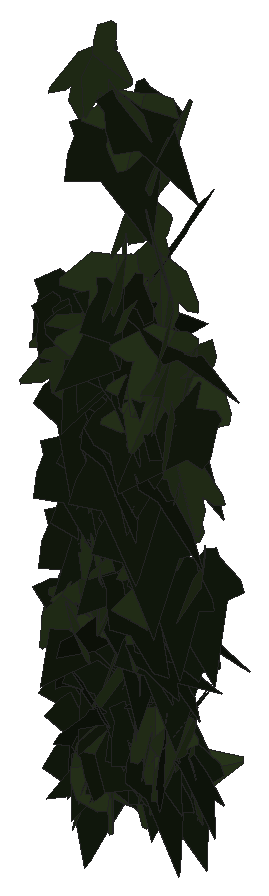
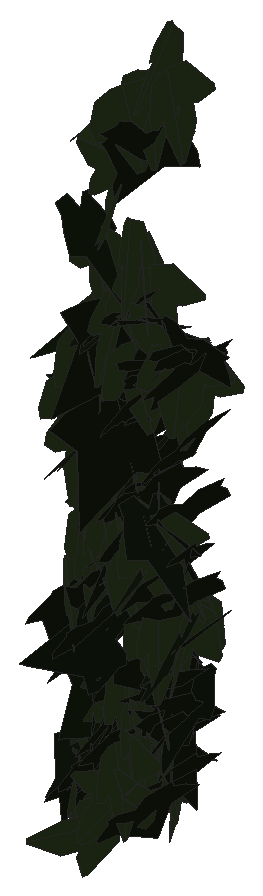
# SketchUp Ruby script. Lengths in inches.
U = 1.inch
M = Sketchup.active_model
def pt(a) = Geom::Point3d.new(a.map { |v| v * U })
def face(e, loops, mat)
  f = e.add_face(loops[0].map { |a| pt(a) })
  loops[1..].each { |l| e.add_face(l.map { |a| pt(a) }).erase! }
  f.material = f.back_material = mat if mat
  f
end
# faces: each face lists its corners as indices into pts; further lists are holes
def faces(e, pts, list, mat = nil) = list.each { |f| face(e, (f[0].is_a?(Array) ? f : [f]).map { |l| l.map { |i| pts[i] } }, mat) }
# xy, xz, yz: faces in a plane at the given z, y or x. An outline is a flat list of corners, or four numbers for a rectangle; further outlines are holes
def ring(l) = l.size == 4 ? [[l[0], l[1]], [l[2], l[1]], [l[2], l[3]], [l[0], l[3]]] : l.each_slice(2).to_a
def flat(e, list, mat, &to3) = list.each { |f| face(e, (f[0].is_a?(Array) ? f : [f]).map { |l| ring(l).map { |u, v| to3.(u, v) } }, mat) }
def xy(e, z, list, mat = nil) = flat(e, list, mat) { |x, y| [x, y, z] }
def xz(e, y, list, mat = nil) = flat(e, list, mat) { |x, z| [x, y, z] }
def yz(e, x, list, mat = nil) = flat(e, list, mat) { |y, z| [x, y, z] }
def lines(e, pts, list) = list.each { |a, b| e.add_line(pt(pts[a]), pt(pts[b])) }
# prism: a flat outline (further loops are holes) pulled along v
def prism(e, loops, v, mat = nil)
  f = face(e, loops, mat); d = Geom::Vector3d.new(v.map { |x| x * U })
  f.pushpull(f.normal.samedirection?(d) ? d.length : -d.length)
end
def box(e, o, s, mat = nil) = prism(e, [[o, [o[0] + s[0], o[1], o[2]], [o[0] + s[0], o[1] + s[1], o[2]], [o[0], o[1] + s[1], o[2]]]], [0, 0, s[2]], mat)
def at(x, y, z, deg = 0) = Geom::Transformation.translation(pt([x, y, z])) * Geom::Transformation.rotation(ORIGIN, Z_AXIS, deg.degrees)
def axes(o, x, y, z) = Geom::Transformation.new([*x, 0, *y, 0, *z, 0, *pt(o).to_a, 1])
def part(name) = M.definitions.add(name)
# library, detail: a bought-in or finely detailed component or shape, given as its bounding box
def library(name, o, s) = part(name).tap { |d| box(d.entities, o, s) }
def detail(e, o, s) = box(e.add_group.entities, o, s)
def put(e, d, t, mat = nil) = e.add_instance(d, t).tap { |i| i.material = mat if mat }
def group(e, t, mat = nil) = e.add_group.tap { |g| g.transformation = t; g.material = mat if mat }.entities
root = M.entities
M.materials.add("efeu1").color = [18, 25, 13]
M.materials.add("efeu2").color = [43, 57, 29]
c1 = part("ivyleaf_9")
p = [[1.54,2.16,1.25],[1.36,2.04,1.19],[-0.21,0.99,0.68],[-0.71,1.11,0.82],[-0.85,0.86,0.67],[-0.8,0.17,0.21],
  [-0.9,-0.01,0.1],[-0.67,-0.16,-0.02],[-0.08,-0.08,-0.05],[-0.03,-0.6,-0.4],[0.65,-0.88,-0.66],[0.83,-0.6,-0.49],
  [1.29,-0.42,-0.43],[1.8125,-0.07,-0.26],[1.21,0.44,0.15]]
faces(c1.entities,p,[[0,1,2,3,4,5,6,7,8,9,10,11,12,13,14]],"efeu1")
c2 = part("ivyleaf_10")
p = [[0,0.5,-0.03],[-0.0625,2.02,-0.43],[-0.19,2.01,-0.46],[-0.54,1.05,-0.29],[-0.52,0.625,-0.18],[-0.83,0.76,-0.28],
  [-1.16,0.64,-0.33],[-1.15,0.33,-0.24],[-0.77,-0.39,0.02],[-0.3,-0.51,0.16],[0.04,-0.48,0.23],[-0.02,2.01,-0.4375],
  [-0.06,2.01,-0.43],[0.04,-0.49,0.23],[0.67,-0.49,0.14],[1.38,0.36,-0.2],[1.375,0.51,-0.24],[0.81,0.65,-0.19],
  [0.62,0.59,-0.15],[0.6,1.09,-0.28],[0.5,1.23,-0.31]]
faces(c2.entities,p,[[0,1,2,3,4,5,6,7,8,9,10],[11,12,0,13,14,15,16,17,18,19,20]],"efeu2")
put(root,c1,axes([23.24,224.17,226.21],[0.01852,-0.47839,-0.14422],[0.05699,0.1454,-0.47499],[0.4964,0.00116,0.05991]))
put(root,c1,axes([23.24,223.85,229.43],[0.14146,-0.43172,-0.20881],[-0.01146,0.2146,-0.45146],[0.47943,0.13252,0.05082]))
put(root,c2,axes([23.55,224.25,227],[-0.25393,-0.41914,0.09918],[-0.03559,-0.09433,-0.48973],[0.42925,-0.25578,0.01808]))
put(root,c2,axes([23.51,223.72,229.37],[-0.33051,-0.37137,-0.05331],[0.03036,0.04434,-0.4971],[0.37395,-0.33184,-0.00676]))
put(root,c1,axes([23.65,224.1875,227.26],[-0.22817,0.42863,-0.11921],[0.05776,-0.1043,-0.48558],[-0.44114,-0.23536,-0.00191]))
put(root,c2,axes([23.59,223.46,225.42],[-0.24049,0.29469,0.32453],[-0.19564,0.2591,-0.38025],[-0.39229,-0.30987,-0.00932]))
put(root,c2,axes([23.53,223.45,229.08],[-0.24872,-0.425,-0.08671],[0.0322,0.08159,-0.49225],[0.43255,-0.25044,-0.01322]))
put(root,c1,axes([23.4,224.75,223.26],[-0.10413,-0.48705,0.04399],[0.00115,-0.04522,-0.49795],[0.48903,-0.1036,0.01054]))
put(root,c2,axes([23.5625,224.08,225.625],[-0.01759,-0.48134,-0.13418],[0.0025,0.13418,-0.48165],[0.49968,-0.01761,-0.00231]))
put(root,c1,axes([23.26,224.1875,225.36],[0.28805,-0.40263,0.07012],[0.04317,-0.05533,-0.49505],[0.4064,0.29125,0.00288]))
put(root,c1,axes([23.37,223.88,227.35],[0.02844,-0.48257,-0.12776],[0.02053,0.12899,-0.48264],[0.49877,0.0222,0.02715]))
put(root,c1,axes([23.49,223.9,225.15],[-0.17656,-0.37444,0.28039],[-0.00324,-0.29872,-0.40095],[0.46778,-0.1434,0.10306]))
put(root,c1,axes([23.4,224.26,226.5],[-0.00186,-0.49802,0.04444],[0.00764,-0.04446,-0.49796],[0.49994,-0.00118,0.00777]))
put(root,c1,axes([23.54,223.38,224.59],[0.4182,-0.00765,-0.27395],[-0.2734,0.02299,-0.418],[0.01899,0.49941,0.01504]))
put(root,c1,axes([23.43,223.9,228.16],[-0.03232,-0.47664,0.14756],[0.01853,-0.14891,-0.47695],[0.49861,-0.02537,0.02729]))
put(root,c1,axes([23.34,223.83,229.78],[-0.18094,-0.25094,-0.3928],[0.35625,0.19726,-0.29013],[0.30057,-0.38486,0.10741]))
put(root,c2,axes([23.53,223.67,225.57],[-0.40171,-0.20217,-0.21854],[0.19322,0.10218,-0.44969],[0.22649,-0.44574,-0.00397]))
put(root,c2,axes([23.55,223.41,225.58],[-0.15429,-0.34275,-0.32972],[0.16956,0.28421,-0.3748],[0.44435,-0.22747,0.02853]))
put(root,c2,axes([23.7,223.66,233.27],[-0.02801,-0.49921,-0.00258],[0.00132,0.00251,-0.49999],[0.49921,-0.02802,0.00118]))
put(root,c2,axes([24.01,223.32,226.09],[-0.16196,0.09948,0.46246],[-0.45935,0.0837,-0.17887],[-0.113,-0.4828,0.06428]))
put(root,c2,axes([23.74,224.69,223.8],[-0.02515,-0.49692,-0.04936],[0.00039,0.04941,-0.49755],[0.49937,-0.02507,-0.0021]))
put(root,c2,axes([23.74,223.79,229.19],[-0.08688,-0.38848,0.30254],[0.04447,-0.31215,-0.38805],[0.49038,-0.04052,0.08879]))
put(root,c1,axes([23.71,223.98,229.24],[-0.24102,-0.43189,0.07332],[-0.01861,-0.07352,-0.49421],[0.43768,-0.24096,0.01937]))
put(root,c2,axes([23.84,223.82,225.56],[-0.26227,-0.37632,0.199],[-0.04535,-0.20771,-0.45255],[0.42327,-0.25543,0.07481]))
put(root,c1,axes([23.7,224.02,224.25],[-0.25181,-0.42707,-0.06482],[0.02996,0.05758,-0.49577],[0.43093,-0.25356,-0.00341]))
put(root,c1,axes([23.77,224.01,229.38],[-0.32089,-0.38306,0.01712],[0.01537,-0.03516,-0.49853],[0.38314,-0.31942,0.03434]))
put(root,c2,axes([23.73,223.85,227.43],[0.22699,-0.4381,-0.0809],[0.05522,0.11776,-0.48279],[0.44207,0.21024,0.10184]))
put(root,c2,axes([23.83,223.42,223.23],[0.15185,-0.37063,-0.29928],[-0.05859,0.2972,-0.39779],[0.47277,0.15588,0.04683]))
put(root,c1,axes([23.93,223.95,226.85],[-0.48859,-0.08267,-0.06669],[0.06554,0.01243,-0.49553],[0.08358,-0.49296,-0.00131]))
put(root,c2,axes([23.8,223.96,224.73],[0.28446,-0.41105,-0.01112],[-0.00679,0.00882,-0.49988],[0.41114,0.28454,-0.00057]))
put(root,c2,axes([23.81,223.8125,223.18],[0.13341,0.08655,0.47404],[-0.11472,0.48343,-0.05597],[-0.46802,-0.09383,0.14885]))
put(root,c1,axes([23.69,223.88,223.18],[-0.07894,-0.48965,0.06333],[0.00504,-0.06493,-0.49574],[0.4937,-0.07763,0.01519]))
put(root,c1,axes([23.66,223.34,224.78],[0.1659,0.17976,0.43607],[0.29169,0.32417,-0.24461],[-0.37067,0.33556,0.00269]))
put(root,c1,axes([23.8,224.16,224.56],[-0.20673,-0.44107,0.11276],[-0.01634,-0.11657,-0.48595],[0.45497,-0.20461,0.03378]))
put(root,c2,axes([23.89,224.18,224.16],[0.07753,-0.484,-0.09867],[0.00047,0.09995,-0.48991],[0.49395,0.07587,0.01595]))
put(root,c1,axes([23.59,224.3125,226.57],[0.23022,-0.43888,0.06621],[0.03144,-0.05827,-0.4956],[0.44273,0.23235,0.00077]))
put(root,c1,axes([23.83,223.92,223.83],[-0.21512,-0.44706,0.06212],[-0.01064,-0.06377,-0.4958],[0.45123,-0.21464,0.01792]))
put(root,c1,axes([23.79,224.1,227.53],[-0.11794,-0.48584,0.00688],[0.00196,-0.00755,-0.49994],[0.48589,-0.1179,0.00369]))
put(root,c2,axes([23.98,224.15,226.4],[-0.0767,-0.44083,0.22313],[-0.02489,-0.22206,-0.44729],[0.49346,-0.07972,0.01212]))
put(root,c2,axes([23.66,224.66,223.37],[0.29172,0.26364,0.30886],[0.22413,0.21259,-0.39316],[-0.33863,0.36783,0.00585]))
put(root,c2,axes([23.97,224.28,224.71],[-0.01009,-0.4981,-0.04237],[0.01138,0.04214,-0.49809],[0.49977,-0.01102,0.01049]))
put(root,c2,axes([24.01,223.98,229.31],[-0.25807,-0.41989,0.08422],[-0.01257,-0.09086,-0.49152],[0.42807,-0.25581,0.03634]))
put(root,c1,axes([24.08,223.54,224.01],[-0.00017,0.39321,-0.30885],[-0.0053,-0.30883,-0.39319],[-0.49997,0.00314,0.00428]))
put(root,c2,axes([23.91,224.13,227.72],[0.27907,-0.41271,0.04229],[0.04637,-0.01962,-0.49746],[0.41227,0.28158,0.02732]))
put(root,c2,axes([23.71,223.86,223.27],[0.30792,-0.18995,0.34511],[0.31552,-0.14336,-0.36041],[0.23587,0.43974,0.03158]))
put(root,c2,axes([24.02,223.74,230.31],[-0.36858,-0.33496,0.04412],[0.03383,-0.10156,-0.48841],[0.33616,-0.35705,0.09754]))
put(root,c2,axes([24.03,224.08,231.12],[0.0932,-0.41518,-0.26257],[-0.02221,0.26342,-0.4244],[0.49073,0.09077,0.03066]))
put(root,c2,axes([23.99,223.2,223.45],[-0.0343,0.1325,0.4809],[-0.07733,0.4748,-0.13633],[-0.49279,-0.08373,-0.01208]))
put(root,c2,axes([24.01,223.9,224.48],[0.12746,-0.47403,0.09514],[0.02879,-0.09078,-0.49085],[0.48262,0.1306,0.00416]))
put(root,c1,axes([23.84,224.36,224.06],[0.07537,-0.44893,-0.20683],[-0.00564,0.20843,-0.45445],[0.49426,0.07083,0.02636]))
put(root,c1,axes([23.86,223.6,223.64],[0.2934,-0.3144,-0.25509],[-0.12723,0.22747,-0.42669],[0.38436,0.31529,0.05348]))
put(root,c1,axes([23.86,224.1,228.92],[0.09447,-0.49093,0.00767],[-0.00018,-0.00784,-0.49994],[0.49099,0.09446,-0.00166]))
put(root,c1,axes([23.98,223.94,224.75],[-0.09591,-0.479,-0.10659],[0.01093,0.1065,-0.4884],[0.49059,-0.09601,-0.00995]))
put(root,c2,axes([24.03,223.65,223.32],[-0.32781,-0.25965,-0.27409],[0.21827,0.16584,-0.41816],[0.30806,-0.3938,0.00462]))
put(root,c2,axes([24.16,223.8,226.19],[0.0415,-0.44989,0.21419],[0.03112,-0.21217,-0.45168],[0.4973,0.05082,0.01039]))
put(root,c2,axes([24.32,223.42,232.91],[-0.46087,0.07978,0.17674],[-0.1806,-0.01064,-0.46612],[-0.07061,-0.49348,0.03863]))
put(root,c2,axes([24.13,223.21,233.59],[0.0896,-0.34457,-0.35106],[0.0812,0.3623,-0.33488],[0.48516,0.003,0.12088]))
put(root,c1,axes([24.03,223.99,226.85],[0.21437,-0.31153,-0.3271],[-0.16297,0.28434,-0.37761],[0.42129,0.26851,0.02037]))
put(root,c2,axes([24.29,223.93,226.08],[-0.3482,-0.24595,0.26127],[-0.07784,-0.30362,-0.38955],[0.35028,-0.31196,0.17315]))
put(root,c1,axes([23.97,223.91,227.49],[0.11248,-0.4692,-0.13115],[-0.00539,0.13339,-0.48185],[0.48715,0.10981,0.02495]))
put(root,c1,axes([24.14,223.99,226.24],[-0.23231,-0.34371,0.2791],[0.00021,-0.31527,-0.38808],[0.44275,-0.1802,0.14663]))
put(root,c2,axes([24.2,223.91,229.82],[0.48066,-0.07552,-0.11518],[-0.10566,0.06604,-0.48423],[0.08835,0.48983,0.04752]))
put(root,c1,axes([24.31,223.87,229.67],[-0.44071,-0.21567,0.09624],[-0.01148,-0.18394,-0.4648],[0.23589,-0.41189,0.15717]))
put(root,c1,axes([23.94,223.81,227.83],[0.14583,-0.45411,0.15006],[0.06354,-0.13709,-0.47662],[0.47402,0.15808,0.01772]))
put(root,c1,axes([24.19,224.11,228.33],[0.2809,0.41354,-0.00892],[-0.01435,-0.00103,-0.49979],[-0.41339,0.28104,0.01129]))
put(root,c2,axes([24.25,223.93,226.66],[0.01185,-0.49961,-0.01576],[-0.00072,0.01575,-0.49975],[0.49986,0.01187,-0.00034]))
put(root,c2,axes([24.27,223.5,230.55],[0.20034,-0.42417,-0.17305],[-0.03189,0.1755,-0.4671],[0.457,0.1982,0.04327]))
put(root,c1,axes([24.53,223.76,223.74],[-0.43822,-0.14146,0.19481],[-0.18555,-0.05934,-0.46049],[0.15341,-0.47588,-0.00049]))
put(root,c1,axes([24.14,223.74,230.02],[-0.28601,-0.08898,-0.40035],[0.40487,0.01656,-0.29293],[0.06539,-0.49174,0.06258]))
put(root,c2,axes([24.08,224.64,222.73],[0.05366,-0.05561,-0.49399],[0.3323,0.37355,-0.00595],[0.36972,-0.32767,0.07705]))
put(root,c1,axes([24.17,223.62,232.38],[-0.15525,-0.34956,-0.32204],[0.14953,0.28566,-0.38215],[0.45115,-0.21496,0.01584]))
put(root,c2,axes([24.35,223.97,226.4375],[0.0325,-0.41575,0.27585],[0.04263,-0.27312,-0.41664],[0.49712,0.0506,0.01769]))
put(root,c1,axes([24.24,224.43,223.59],[-0.10638,-0.48793,-0.02474],[-0.0038,0.02615,-0.4993],[0.48854,-0.10604,-0.00927]))
put(root,c1,axes([24.16,224.2,223.6],[0.09707,-0.48997,-0.02253],[-0.00065,0.02284,-0.49948],[0.49049,0.097,0.00379]))
put(root,c2,axes([24.37,223.89,229.89],[-0.08829,-0.42866,-0.24178],[0.07065,0.23206,-0.43722],[0.48705,-0.11137,0.01959]))
put(root,c1,axes([24.28,224,228.15],[-0.14947,-0.47658,-0.02298],[0.01033,0.02084,-0.49946],[0.47702,-0.14978,0.00361]))
put(root,c1,axes([24.24,223.87,229.87],[-0.04873,-0.49009,-0.08624],[-0.0063,0.08725,-0.49229],[0.49758,-0.04689,-0.01468]))
put(root,c2,axes([24.45,223.67,232.78],[-0.30635,-0.37679,0.11909],[0.00679,-0.15569,-0.47509],[0.3951,-0.28947,0.10051]))
put(root,c1,axes([24.15,223.92,224.88],[0.10954,-0.37741,0.30913],[0.06606,-0.30244,-0.39264],[0.48336,0.12686,-0.0164]))
put(root,c2,axes([24.41,223.59,224.59],[0.34813,-0.33039,-0.14019],[-0.02456,0.17291,-0.46851],[0.35806,0.33309,0.10416]))
put(root,c1,axes([24.24,223.9,229.59],[0.44008,0.23177,0.05106],[0.05112,0.01247,-0.49722],[-0.23176,0.44286,-0.01272]))
put(root,c2,axes([24.35,223.93,227.21],[0.2179,-0.43115,0.12895],[0.12109,-0.08181,-0.47817],[0.43343,0.23961,0.06877]))
put(root,c1,axes([24.33,223.6,227.66],[-0.09631,-0.46525,-0.15579],[0.02268,0.15437,-0.47503],[0.49011,-0.09856,-0.00863]))
put(root,c1,axes([24.32,224.49,225.59],[-0.04446,-0.49758,0.021],[0.00026,-0.0211,-0.49955],[0.49802,-0.04441,0.00213]))
put(root,c2,axes([24.36,224.01,223.18],[0.07267,-0.30364,-0.39054],[0.17352,0.3853,-0.26727],[0.46326,-0.09669,0.16137]))
put(root,c2,axes([24.59,224.01,226.82],[-0.28069,-0.39403,0.12631],[-0.07023,-0.10505,-0.48377],[0.40778,-0.28932,0.00363]))
put(root,c2,axes([24.51,223.74,223.71],[0.24079,-0.37858,-0.22066],[-0.0224,0.24082,-0.43761],[0.43763,0.22063,0.09902]))
put(root,c2,axes([24.57,223.9,228.37],[-0.34398,-0.34558,0.11067],[-0.01194,-0.14163,-0.47937],[0.36267,-0.33244,0.08918]))
put(root,c1,axes([24.13,224.39,225.36],[0.44053,-0.14041,0.1903],[0.18432,-0.04826,-0.46228],[0.14818,0.47745,0.00924]))
put(root,c1,axes([24.35,223.93,223.95],[0.14448,-0.45544,-0.14732],[-0.04479,0.14034,-0.47781],[0.47657,0.15126,-0.00024]))
put(root,c1,axes([24.38,224.01,225.43],[0.273,-0.41471,-0.05904],[-0.02451,0.05454,-0.49641],[0.41817,0.27394,0.00945]))
put(root,c1,axes([24.4,223.57,225.89],[0.24376,-0.43616,-0.01861],[-0.00775,0.01699,-0.49965],[0.43649,0.24388,0.00152]))
put(root,c1,axes([24.37,224.06,227.45],[0.2769,-0.40424,0.09958],[0.07266,-0.07083,-0.4896],[0.40994,0.2856,0.01952]))
put(root,c2,axes([24.7,224.04,226.41],[0.04521,-0.48368,-0.11838],[0.02277,0.12075,-0.48467],[0.49743,0.03843,0.03294]))
put(root,c2,axes([24.71,223.7,231.96],[0.18501,-0.28576,0.36622],[-0.15332,0.33454,0.33849],[-0.43848,-0.23754,0.03616]))
put(root,c1,axes([24.48,224.27,223.29],[0.07833,-0.46694,-0.16074],[0.01479,0.16489,-0.4718],[0.49361,0.06915,0.03964]))
put(root,c2,axes([24.68,223.65,225.95],[-0.03751,-0.47135,0.16254],[0.07165,-0.16641,-0.46602],[0.49342,-0.01167,0.08003]))
put(root,c2,axes([24.71,224.28,227.74],[0.24659,-0.41562,-0.12827],[-0.01388,0.13986,-0.47984],[0.43474,0.24021,0.05744]))
put(root,c2,axes([24.625,223.78,223.98],[0.04614,0.47955,-0.13379],[-0.00483,-0.13392,-0.48171],[-0.49784,0.04575,-0.00773]))
put(root,c2,axes([24.79,223.72,230.59],[-0.48495,0.10924,0.05378],[-0.07078,-0.07319,-0.48952],[-0.09908,-0.4824,0.08645]))
put(root,c2,axes([24.78,223.67,229.03],[-0.16778,-0.42491,0.20322],[-0.0146,-0.21093,-0.45309],[0.47078,-0.15797,0.05837]))
put(root,c1,axes([24.45,223.56,232.9],[0.2408,-0.41859,-0.1296],[0.0425,0.16949,-0.46847],[0.43613,0.2146,0.11721]))
put(root,c2,axes([24.78,224.33,223.11],[-0.30779,0.39314,0.02658],[-0.08526,-0.03351,-0.49154],[-0.38471,-0.30711,0.08767]))
put(root,c1,axes([24.6,223.64,226.97],[-0.0342,-0.49104,-0.08781],[0.00064,0.08798,-0.4922],[0.49883,-0.03378,-0.00539]))
put(root,c1,axes([24.96,223.93,231.12],[-0.2908,0.39639,-0.09115],[0.05296,-0.07419,-0.49162],[-0.40327,-0.29558,0.00116]))
put(root,c2,axes([24.73,223.61,231.22],[-0.25824,0.42814,-0.00324],[0.0016,-0.00282,-0.49999],[-0.42815,-0.25824,0.00008]))
put(root,c2,axes([24.74,223.94,229.16],[0.23756,-0.42918,0.09681],[0.04369,-0.08646,-0.49053],[0.43779,0.24152,-0.00358]))
put(root,c1,axes([24.51,224.16,228.23],[0.26243,-0.41513,-0.0938],[0.00364,0.11239,-0.48719],[0.42558,0.25502,0.06201]))
put(root,c1,axes([24.96,223.52,223.96],[0.02095,0.0111,-0.49944],[-0.44053,0.23612,-0.01324],[0.23556,0.44059,0.01968]))
put(root,c1,axes([24.64,224.06,225.18],[-0.04219,-0.49222,-0.07705],[0.00913,0.07655,-0.49402],[0.49813,-0.0431,0.00252]))
put(root,c1,axes([24.64,223.42,225.31],[0.45056,-0.04246,-0.21258],[-0.16788,0.24188,-0.40412],[0.13716,0.43553,0.20371]))
put(root,c2,axes([24.89,223.64,229.58],[-0.21805,-0.38996,0.22446],[-0.03901,-0.23211,-0.44114],[0.44825,-0.20989,0.0708]))
put(root,c2,axes([24.83,223.77,228.56],[0.24097,-0.35052,-0.26281],[-0.02743,0.28729,-0.40831],[0.43724,0.2112,0.11923]))
put(root,c1,axes([24.64,224.46,225.93],[0.01683,-0.47152,-0.1655],[-0.00311,0.16549,-0.47181],[0.49971,0.01691,0.00264]))
put(root,c1,axes([24.89,223.59,223.9],[0.12936,0.276,0.39634],[0.007,0.4092,-0.28724],[-0.48292,0.07986,0.10201]))
put(root,c2,axes([24.86,224.3,225.98],[0.18485,-0.45093,-0.11175],[-0.00427,0.11862,-0.48571],[0.46455,0.18052,0.04]))
put(root,c2,axes([24.875,224.1,228.7],[-0.3822,-0.30463,0.10547],[0.03709,-0.20405,-0.45496],[0.32023,-0.33995,0.17858]))
put(root,c1,axes([25.04,223.96,228.57],[-0.4919,-0.08897,-0.01096],[0.01172,-0.00322,-0.49985],[0.08887,-0.49201,0.00525]))
put(root,c1,axes([24.62,223.8,223.36],[0.16862,-0.45201,0.13135],[0.04224,-0.12443,-0.48242],[0.46881,0.17379,-0.00377]))
put(root,c1,axes([24.68,224.04,226.14],[0.06418,-0.49047,0.07293],[0.01803,-0.07118,-0.49458],[0.49554,0.06611,0.00855]))
put(root,c1,axes([24.59,223.77,229.78],[0.40396,-0.28812,-0.06171],[0.03301,0.14831,-0.47636],[0.2928,0.38078,0.13884]))
put(root,c2,axes([24.95,223.99,229.2],[-0.07766,-0.49393,0.00002],[-0.00182,0.00026,-0.5],[0.49393,-0.07766,-0.00184]))
put(root,c2,axes([24.89,223.92,223.88],[0.09542,-0.38439,0.30519],[0.1105,-0.2861,-0.39489],[0.47821,0.14281,0.03035]))
put(root,c2,axes([25.03,223.77,227.8],[-0.49805,0.04291,0.01031],[-0.01021,0.00164,-0.49989],[-0.04293,-0.49815,-0.00076]))
put(root,c1,axes([24.69,224.32,223.36],[0.15034,-0.38267,0.28453],[0.14489,-0.24758,-0.40953],[0.45432,0.20559,0.03645]))
put(root,c2,axes([25.05,223.44,230.04],[0.24999,-0.40017,-0.16544],[-0.05175,0.16205,-0.47017],[0.42991,0.2522,0.03961]))
